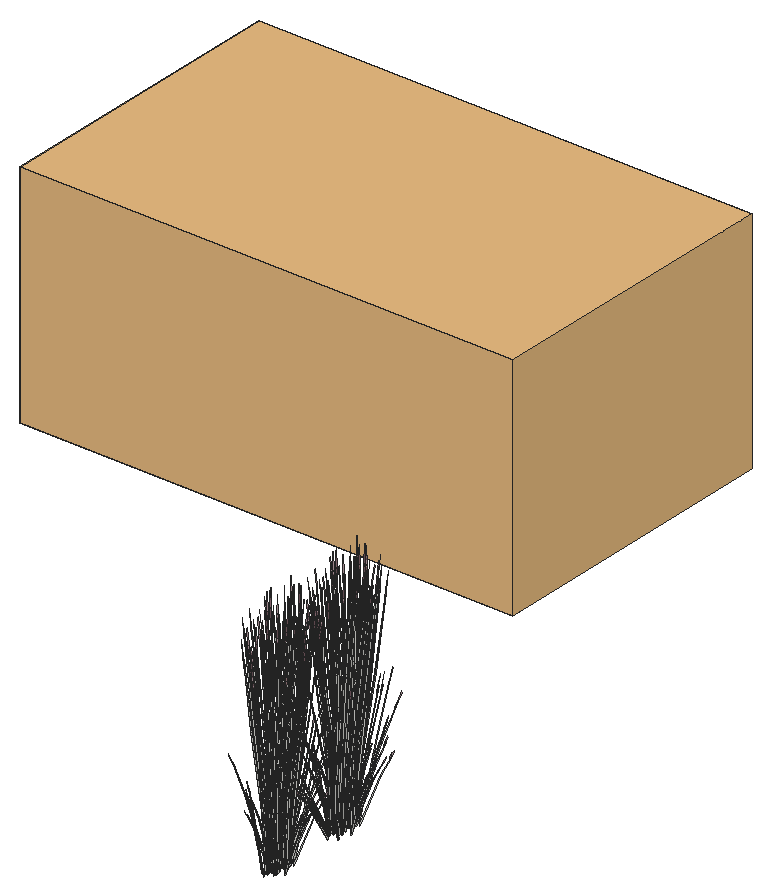
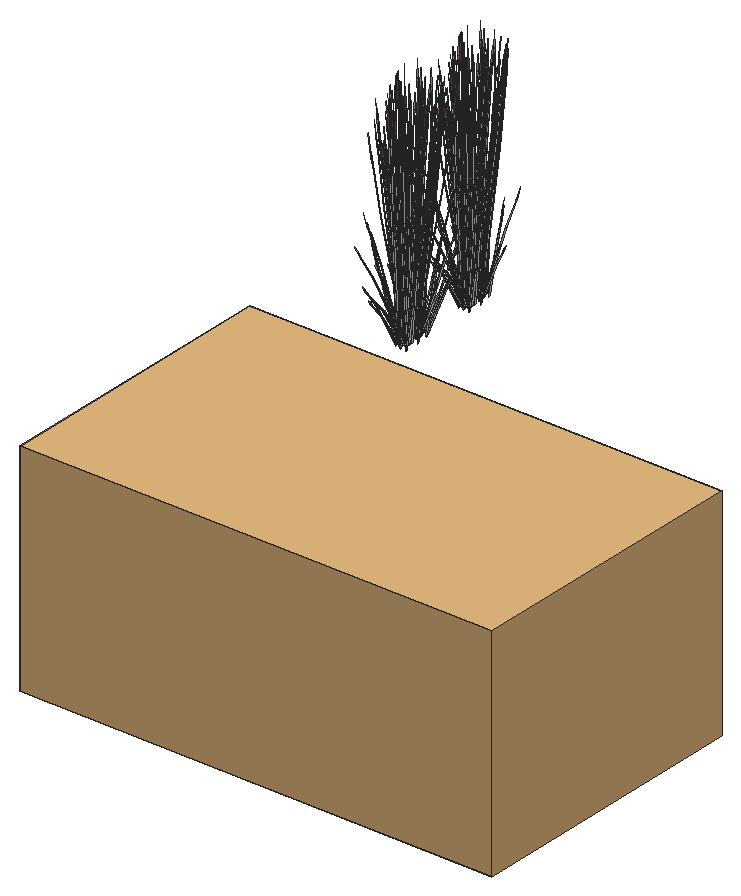
# SketchUp Ruby script. Lengths in inches.
U = 1.inch
M = Sketchup.active_model
def pt(a) = Geom::Point3d.new(a.map { |v| v * U })
def face(e, loops, mat)
  f = e.add_face(loops[0].map { |a| pt(a) })
  loops[1..].each { |l| e.add_face(l.map { |a| pt(a) }).erase! }
  f.material = f.back_material = mat if mat
  f
end
# faces: each face lists its corners as indices into pts; further lists are holes
def faces(e, pts, list, mat = nil) = list.each { |f| face(e, (f[0].is_a?(Array) ? f : [f]).map { |l| l.map { |i| pts[i] } }, mat) }
# xy, xz, yz: faces in a plane at the given z, y or x. An outline is a flat list of corners, or four numbers for a rectangle; further outlines are holes
def ring(l) = l.size == 4 ? [[l[0], l[1]], [l[2], l[1]], [l[2], l[3]], [l[0], l[3]]] : l.each_slice(2).to_a
def flat(e, list, mat, &to3) = list.each { |f| face(e, (f[0].is_a?(Array) ? f : [f]).map { |l| ring(l).map { |u, v| to3.(u, v) } }, mat) }
def xy(e, z, list, mat = nil) = flat(e, list, mat) { |x, y| [x, y, z] }
def xz(e, y, list, mat = nil) = flat(e, list, mat) { |x, z| [x, y, z] }
def yz(e, x, list, mat = nil) = flat(e, list, mat) { |y, z| [x, y, z] }
def lines(e, pts, list) = list.each { |a, b| e.add_line(pt(pts[a]), pt(pts[b])) }
# prism: a flat outline (further loops are holes) pulled along v
def prism(e, loops, v, mat = nil)
  f = face(e, loops, mat); d = Geom::Vector3d.new(v.map { |x| x * U })
  f.pushpull(f.normal.samedirection?(d) ? d.length : -d.length)
end
def box(e, o, s, mat = nil) = prism(e, [[o, [o[0] + s[0], o[1], o[2]], [o[0] + s[0], o[1] + s[1], o[2]], [o[0], o[1] + s[1], o[2]]]], [0, 0, s[2]], mat)
def at(x, y, z, deg = 0) = Geom::Transformation.translation(pt([x, y, z])) * Geom::Transformation.rotation(ORIGIN, Z_AXIS, deg.degrees)
def axes(o, x, y, z) = Geom::Transformation.new([*x, 0, *y, 0, *z, 0, *pt(o).to_a, 1])
def part(name) = M.definitions.add(name)
# library, detail: a bought-in or finely detailed component or shape, given as its bounding box
def library(name, o, s) = part(name).tap { |d| box(d.entities, o, s) }
def detail(e, o, s) = box(e.add_group.entities, o, s)
def put(e, d, t, mat = nil) = e.add_instance(d, t).tap { |i| i.material = mat if mat }
def group(e, t, mat = nil) = e.add_group.tap { |g| g.transformation = t; g.material = mat if mat }.entities
root = M.entities
M.materials.add("LightPink_Translucent").color = [144, 107, 117]
M.materials["LightPink_Translucent"].alpha = 0.75
c1 = part("blade")
p = [[2.15,0.21,22],[0,0.17,0],[0.09,0.45,0],[2.18,0.31,22],[2.29,0.31,22],[0.38,0.45,0],
  [2.48,0.24,33],[2.49,0.24,33],[2.48,0.22,33]]
faces(c1.entities,p,[[0,1,2,3],[4,5,2,3],[6,3,4,7],[8,0,3,6]])
c2 = part("seeds")
p = [[0.3,-0.1,1.38],[-0.01,-0.03,1.59],[-0.01,-0.03,0.03],[0.14,-0.07,-0.07],[0.29,-0.03,3],[0.15,0.01,3.11]]
faces(c2.entities,p,[[0,1,2,3],[1,0,4,5]],"LightPink_Translucent")
c3 = part("blade with seeds")
put(c3.entities,c1,at(0,0,0))
put(c3.entities,c2,axes([2.4,0.25,30.99],[1.5799,-0.05474,1.17369],[-0.12525,1.92788,0.29478],[-0.07173,-0.02425,1.56792]))
c4 = library("2016+Honda+Civic+LX+Sedan",[0.01,0.03,0.02],[16.17,34.46,10.62])
put(root,c3,axes([251.21,225.6,0.91],[-0.16003,-0.61271,0],[0.26773,-0.34169,-0.37456],[0.06098,-0.07782,1.18819]))
put(root,c3,axes([251.56,224.86,0.74],[-0.17688,0.35078,-0.02825],[-0.16207,-0.38418,-0.1281],[-0.01141,-0.10886,0.42251]))
put(root,c3,axes([250.64,227.32,0.66],[0,-0.61145,-0.36036],[0.28637,0,0],[0,-0.13926,1.14313]))
put(root,c3,axes([251.43,225.51,0.66],[0.23955,-0.30573,-0.36036],[0.14318,0.54821,0],[0.05456,-0.06963,1.14313]))
put(root,c3,axes([252.85,226.5625,1.07],[-0.09144,-0.01811,1.03788],[-0.09368,-0.48584,-0.22321],[0.11233,-0.13744,0.44375]))
put(root,c3,axes([251.71,226.76,0.6875],[0.1724,-0.45959,-0.45255],[0.21416,0.41674,-0.11877],[0.06908,-0.11465,0.99892]))
put(root,c3,axes([252.96,225.67,1.2],[-0.08525,0.31126,0.83364],[-0.07328,-0.41819,0.6125],[0.07041,-0.10479,0.18362]))
put(root,c3,axes([251.41,227.57,0.8],[0.12419,-0.55096,-0.32471],[0.25804,0.26516,0.15627],[0,-0.12701,1.04254]))
put(root,c3,axes([251.53,227.29,1.13],[-0.02983,-0.6977,-0.21117],[0.31064,-0.04219,-0.36291],[0.0547,-0.09294,1.15913]))
put(root,c3,axes([250.76,227.33,0.66],[0.17867,-0.3815,-0.22483],[0.17867,0.3815,0.22483],[0,-0.12288,1.00865]))
put(root,c3,axes([250.6875,225.5,0.74],[-0.07384,0.49928,-0.02825],[-0.22725,-0.15358,-0.1281],[-0.0345,-0.08166,0.42251]))
put(root,c3,axes([251.38,228.02,1.13],[-0.28825,-0.29175,-0.21117],[0.1388,-0.61578,-0.36291],[-0.00906,-0.15119,1.15913]))
put(root,c3,axes([250.5625,227.78,0.91],[-0.32006,0,0],[0,-0.68339,-0.37456],[0,-0.15565,1.18819]))
put(root,c3,axes([250.62,226.56,1.07],[0.04997,0.17024,1.03788],[-0.11515,0.46273,-0.22321],[-0.11824,-0.1106,0.44375]))
put(root,c3,axes([251.49,225.75,0.66],[0.23879,0.15129,-0.22483],[-0.06012,0.53279,0.22483],[0.04814,-0.06144,1.00865]))
put(root,c3,axes([250.8125,227.6,0.88],[-0.23808,0.51407,0.22322],[-0.23822,-0.50866,-0.26485],[-0.00831,-0.14599,1.19671]))
put(root,c3,axes([251.57,227.84,0.96],[0.28839,0.29636,0.17466],[-0.1388,0.61578,0.36291],[0,-0.14195,1.16519]))
put(root,c3,axes([251.46,228.67,0.96],[0.06784,-0.72454,-0.17004],[0.32166,0.1263,0.37211],[-0.05621,-0.10006,1.13542]))
put(root,c3,axes([250.32,227.07,1.2],[0.16341,-0.04375,0.83364],[-0.10366,0.38551,0.6125],[-0.08075,-0.05783,0.18362]))
put(root,c3,axes([251.48,227.43,1.17],[-0.27795,0.03775,0.32471],[-0.02514,-0.62656,-0.15627],[0.04976,-0.0635,1.04254]))
put(root,c3,axes([250.76,227.88,0.99],[0,0.61145,0.36036],[-0.28637,0,0],[0,-0.13926,1.14313]))
put(root,c3,axes([252.39,225.76,0.92],[0.16003,-0.61271,0],[0.26773,0.34169,-0.37456],[0.06098,0.07782,1.18819]))
put(root,c3,axes([251.43,228.375,0.8],[-0.15376,-0.51322,-0.32471],[0.2329,-0.3614,0.15627],[-0.04976,-0.0635,1.04254]))
put(root,c3,axes([251.47,227.65,0.91],[0.11128,0.68373,0.33208],[-0.31797,0.23776,0.13031],[0.00389,-0.12563,1.15295]))
put(root,c3,axes([253.02,228.18,0.63],[-0.16485,0.07338,1.02759],[-0.02624,-0.58408,0.05882],[0.11546,-0.08841,0.58473]))
put(root,c3,axes([253.32,227.66,0.83],[-0.15869,-0.39099,-0.04709],[0.1738,-0.35825,-0.21349],[0.04925,-0.02522,0.70419]))
put(root,c3,axes([251.41,228.19,1.17],[-0.12419,0.55096,0.32471],[-0.25804,-0.26516,-0.15627],[0,-0.12701,1.04254]))
put(root,c3,axes([251.87,227.71,0.79],[0,-0.70749,0],[0.32006,0,0],[0,0,1.30246]))
put(root,c3,axes([252.25,226.08,0.99],[-0.23955,-0.30573,0.36036],[0.14318,-0.54821,0],[0.05456,0.06963,1.14313]))
put(root,c3,axes([251.3,228.57,0.6875],[-0.26625,-0.10025,-0.45255],[0.05619,-0.61836,-0.11877],[-0.07946,-0.07493,0.99892]))
put(root,c3,axes([251.71,227.26,0.91],[-0.21222,0.5549,0.33208],[-0.25213,-0.48983,0.13031],[0.05116,-0.05538,1.15295]))
put(root,c3,axes([251.95,228.26,0.86],[-0.23808,-0.52628,-0.0445],[0.23822,-0.5266,0],[-0.00831,-0.01838,1.27426]))
put(root,c3,axes([251.35,226.35,0.99],[-0.07394,0.60768,0.12804],[-0.27057,-0.17197,0.25465],[0.04674,-0.00296,1.1642]))
put(root,c3,axes([251.23,226.84,0.35],[-0.25194,0.2448,0.93574],[-0.08019,-0.7024,0.36359],[0.1547,0.01169,1.0643]))
put(root,c3,axes([251.91,227.03,1.09],[0.04938,-0.54569,0.10509],[0.24125,0.09472,-0.30009],[0.0439,0.05603,0.91989]))
put(root,c3,axes([251.49,228.32,0.91],[0.32351,0.12883,0.33208],[-0.06584,0.72759,0.13031],[-0.04728,-0.07026,1.15295]))
put(root,c3,axes([253.2,227.79,0.28],[-0.01338,-0.09283,1.27986],[0.09278,-0.54301,-0.19552],[0.09359,-0.00781,0.218]))
put(root,c3,axes([250.44,227.7,0.28],[0.00649,0.09636,1.27986],[-0.13086,0.50324,-0.19552],[-0.09295,-0.02537,0.218]))
put(root,c3,axes([251.81,227.17,1.17],[-0.15376,-0.51322,0.32471],[0.2329,-0.3614,-0.15627],[0.04976,0.0635,1.04254]))
put(root,c3,axes([251.01,229.52,0.66],[-0.06012,-0.53279,-0.22483],[0.23879,-0.15129,0.22483],[-0.04814,-0.06144,1.00865]))
put(root,c3,axes([251.32,229.48,0.99],[0.27504,-0.16229,0.12804],[0.06792,0.60396,0.25465],[-0.02453,-0.088,1.1642]))
put(root,c3,axes([251.89,227.2,1.13],[0.25843,-0.40595,-0.21117],[0.17185,0.5736,-0.36291],[0.06376,0.05825,1.15913]))
put(root,c3,axes([250.95,229.74,0.66],[-0.23955,-0.30573,-0.36036],[0.14318,-0.54821,0],[-0.05456,-0.06963,1.14313]))
put(root,c3,axes([252.54,226.125,0.66],[0.23955,0.30573,-0.36036],[-0.14318,0.54821,0],[0.05456,0.06963,1.14313]))
put(root,c3,axes([252.08,227.87,0.79],[0.28637,0,0],[0,0.63302,0],[0,0,1.29484]))
put(root,c3,axes([251.6,228.66,1.13],[-0.25843,0.40595,-0.21117],[-0.17185,-0.5736,-0.36291],[-0.06376,-0.05825,1.15913]))
put(root,c3,axes([252.16,226.38,0.99],[-0.27504,0.16229,0.12804],[-0.06792,-0.60396,0.25465],[0.02453,0.088,1.1642]))
put(root,c3,axes([252.47,226.35,0.66],[0.06012,0.53279,-0.22483],[-0.23879,0.15129,0.22483],[0.04814,0.06144,1.00865]))
put(root,c3,axes([251.99,227.55,0.92],[-0.32351,-0.12883,0.35707],[0.06584,-0.72759,0.14012],[0.04728,0.07026,1.23973]))
put(root,c3,axes([251.73,229.34,0.79],[-0.08351,-0.52716,0],[0.23848,-0.18461,0],[0,0,1.1204]))
put(root,c3,axes([251.57,228.84,1.09],[-0.04938,0.54569,0.10509],[-0.24125,-0.09472,-0.30009],[-0.0439,-0.05603,0.91989]))
put(root,c3,axes([252.05,229.27,0.78],[0.26872,-0.20746,-0.13933],[0.09442,0.59762,0.00006],[0.02966,-0.02293,1.26212]))
put(root,c3,axes([252.14,229.52,0.99],[0.07394,-0.60768,0.12804],[0.27057,0.17197,0.25465],[-0.04674,0.00296,1.1642]))
put(root,c3,axes([252.08,228.14,0.8],[0.17867,0.39495,0],[-0.17867,0.39495,0],[0,0,1.22851]))
put(root,c3,axes([252.5625,227.97,0.99],[-0.2011,-0.44539,0.12804],[0.20266,-0.432,0.25465],[-0.02221,0.09096,1.1642]))
put(root,c3,axes([252.1875,227.29,0.6875],[0.26625,0.10025,-0.45255],[-0.05619,0.61836,-0.11877],[0.07946,0.07493,0.99892]))
put(root,c3,axes([253.36,228.375,1.2],[-0.15814,0.10094,0.83364],[0.07444,-0.41719,0.6125],[0.0839,0.02855,0.18362]))
put(root,c3,axes([251.67,229.58,0.79],[-0.25804,-0.27452,0],[0.12419,-0.5704,0],[0,0,1.1809]))
put(root,c3,axes([251.89,228.85,0.98],[-0.24993,-0.49214,-0.18284],[0.21031,-0.55263,0.40012],[-0.0673,0.05757,1.22088]))
put(root,c3,axes([251.23,229.79,0.99],[0.23955,0.30573,0.36036],[-0.14318,0.54821,0],[-0.05456,-0.06963,1.14313]))
put(root,c3,axes([252.07,227.68,1.17],[0.12419,-0.55096,0.32471],[0.25804,0.26516,-0.15627],[0,0.12701,1.04254]))
put(root,c3,axes([252.03,227.99,0.86],[0,0.70714,-0.04091],[-0.32006,0,0],[0,0.02222,1.30182]))
put(root,c3,axes([252.05,227.49,0.8],[0.15376,0.51322,-0.32471],[-0.2329,0.3614,0.15627],[0.04976,0.0635,1.04254]))
put(root,c3,axes([251.09,230.11,0.91],[-0.16003,0.61271,0],[-0.26773,-0.34169,-0.37456],[-0.06098,-0.07782,1.18819]))
put(root,c3,axes([252.73,227.98,0.99],[0,-0.61145,0.36036],[0.28637,0,0],[0,0.13926,1.14313]))
put(root,c3,axes([252.01,228.44,1.17],[0.27795,-0.03775,0.32471],[0.02514,0.62656,-0.15627],[-0.04976,0.0635,1.04254]))
put(root,c3,axes([252.18,227.8,1.09],[0.23848,-0.17832,0.10509],[0.08351,0.5092,-0.30009],[0,0.11207,0.91989]))
put(root,c3,axes([251.76,228.75,0.8],[-0.27795,0.03775,-0.32471],[-0.02514,-0.62656,0.15627],[-0.04976,0.0635,1.04254]))
put(root,c3,axes([253.07,229.04,1.07],[-0.06164,-0.15038,1.03788],[0.0802,-0.49748,-0.22321],[0.12472,0.06739,0.44375]))
put(root,c3,axes([251.97,229.59,0.79],[0.25804,0.27452,0],[-0.12419,0.5704,0],[0,0,1.26978]))
put(root,c3,axes([252.07,230.2,0.78],[-0.15803,-0.61485,-0.03732],[0.26773,-0.34169,0.37456],[-0.06597,0.05854,1.1876]))
put(root,c3,axes([252.01,228.71,1.09],[0.1891,0.36737,0.10509],[-0.15773,0.41447,-0.30009],[-0.0439,0.05603,0.91989]))
put(root,c3,axes([252.21,229.84,0.99],[0.23955,-0.30573,0.36036],[0.14318,0.54821,0],[-0.05456,0.06963,1.14313]))
put(root,c3,axes([251.875,229.36,0.86],[0.11128,0.70245,-0.04364],[-0.31797,0.24614,0],[0.00389,0.02453,1.2496]))
put(root,c3,axes([252,230.12,0.66],[-0.23879,-0.15129,-0.22483],[0.06012,-0.53279,0.22483],[-0.04814,0.06144,1.00865]))
put(root,c3,axes([250.27,229.04,1.07],[0.08895,0.05019,1.03788],[0.05733,0.5127,-0.22321],[-0.12083,0.09597,0.44375]))
put(root,c3,axes([252.92,228.09,0.92],[0.32006,0,0],[0,0.68339,-0.37456],[0,0.15565,1.18819]))
put(root,c3,axes([252.79,228.4375,0.79],[-0.3199,-0.00489,-0.03612],[0,-0.68339,0.36248],[-0.01005,0.15557,1.14929]))
put(root,c3,axes([252.1,227.84,1.13],[0.28825,0.29175,-0.21117],[-0.1388,0.61578,-0.36291],[0.00906,0.15119,1.15913]))
put(root,c3,axes([250.09,230.11,1.2],[0.10667,-0.27712,0.83364],[0.04209,0.43871,0.6125],[-0.07709,0.07855,0.18362]))
put(root,c3,axes([252.73,228.54,0.66],[-0.17867,0.3815,-0.22483],[-0.17867,-0.3815,0.22483],[0,0.12288,1.00865]))
put(root,c3,axes([251.96,228.58,1.13],[0.02983,0.6977,-0.21117],[-0.31064,0.04219,-0.36291],[-0.0547,0.09294,1.15913]))
put(root,c3,axes([252.07,228.3,0.8],[-0.12419,0.55096,-0.32471],[-0.25804,-0.26516,0.15627],[0,0.12701,1.04254]))
put(root,c3,axes([251.77,229.11,0.6875],[-0.1724,0.45959,-0.45255],[-0.21416,-0.41674,-0.11877],[-0.06908,0.11465,0.99892]))
put(root,c3,axes([252.08,229.88,0.88],[0.32044,0.19874,0.22322],[-0.08017,0.71038,-0.26485],[-0.05304,0.08891,1.19671]))
put(root,c3,axes([252.05,230.36,0.66],[-0.23955,0.30573,-0.36036],[-0.14318,-0.54821,0],[-0.05456,0.06963,1.14313]))
put(root,c3,axes([252.85,228.55,0.66],[0,0.61145,-0.36036],[-0.28637,0,0],[0,0.13926,1.14313]))
put(root,c3,axes([252.49,229.82,1.2],[-0.14411,-0.17581,0.83364],[0.18609,-0.17864,0.6125],[0.05019,0.15132,0.18362]))
put(root,c3,axes([252.27,230.27,0.91],[0.16003,0.61271,0],[-0.26773,0.34169,-0.37456],[-0.06098,0.07782,1.18819]))
put(root,c3,axes([252.53,230.47,0.28],[0.01865,-0.08828,1.27986],[0.23477,-0.25998,-0.19552],[0.07118,0.13456,0.218]))
put(root,c3,axes([252.13,227.84,1.26],[-0.00699,-0.5757,1.02533],[0.31645,0.14923,0.43413],[-0.07484,0.31502,0.96783]))
put(root,c3,axes([252.22,228.47,0.71],[0.09385,0.55983,-0.50233],[-0.27035,0.20162,-0.13184],[0.01037,0.18957,1.1088]))
put(root,c3,axes([250.37,230.4,0.28],[0.03433,0.06109,1.27986],[0.05822,0.56601,-0.19552],[-0.07609,0.1207,0.218]))
put(root,c3,axes([252.51,230.62,1.13],[-0.16414,-0.01918,0.76251],[0.10839,-0.40729,0.421],[0.06484,0.1447,0.59812]))
put(root,c3,axes([251.97,229.63,1.07],[0.00452,-0.20269,1.03788],[0.21585,-0.22641,-0.22321],[0.06663,0.2426,0.44375]))
put(root,c3,axes([250.99,231.32,1.2],[-0.00662,-0.36357,0.83364],[0.16552,0.25931,0.6125],[-0.03255,0.17329,0.18362]))
put(root,c3,axes([251.43,230.45,0.28],[0.04142,-0.03327,1.27986],[0.24917,0.18313,-0.19552],[0.00729,0.2064,0.218]))
put(root,c3,axes([250.86,230.54,1.24],[0.23252,-0.10828,0.04723],[0.05346,0.43623,-0.62638],[-0.01474,0.22082,0.56147]))
put(root,c3,axes([252.15,240.19,1.07],[-0.07276,0.12376,1.03788],[-0.21789,-0.21662,-0.22321],[0.04039,-0.2694,0.44375]))
put(root,c3,axes([250.8,231,1.07],[0.08077,-0.09646,1.03788],[0.19942,0.29084,-0.22321],[-0.05936,0.25166,0.44375]))
put(root,c3,axes([251.03,239.96,1.07],[-0.0155,0.20002,1.03788],[-0.22659,0.16744,-0.22321],[-0.05297,-0.25854,0.44375]))
put(root,c3,axes([251.61,239.52,0.28],[-0.04293,0.02203,1.27986],[-0.23742,-0.24798,-0.19552],[0.00398,-0.20684,0.218]))
put(root,c3,axes([251.88,239.2,1.2],[0.03283,0.35655,0.83364],[-0.18215,-0.19748,0.6125],[0.0196,-0.18257,0.18362]))
put(root,c3,axes([250.95,239.63,1.2],[0.13352,0.21281,0.83364],[-0.19445,0.12793,0.6125],[-0.0416,-0.16355,0.18362]))
put(root,c3,axes([250.84,240.27,0.28],[-0.02479,0.08055,1.27986],[-0.25056,0.17367,-0.19552],[-0.06053,-0.15798,0.218]))
put(root,c3,axes([251.25,242.49,0.72],[-0.10512,-0.62701,-0.50685],[0.30279,-0.22582,-0.13303],[-0.01162,-0.21232,1.11879]))
put(root,c3,axes([252.66,240.57,0.28],[-0.03831,-0.04817,1.27986],[-0.0984,-0.53815,-0.19552],[0.06638,-0.14604,0.218]))
put(root,c3,axes([251.21,240.69,0.91],[-0.16003,-0.61271,0],[0.26773,-0.34169,-0.37456],[0.06098,-0.07782,1.18819]))
put(root,c3,axes([251.56,239.95,0.74],[-0.17688,0.35078,-0.02825],[-0.16207,-0.38418,-0.1281],[-0.01141,-0.10886,0.42251]))
put(root,c3,axes([250.64,242.4,0.66],[0,-0.61145,-0.36036],[0.28637,0,0],[0,-0.13926,1.14313]))
put(root,c3,axes([251.43,240.59,0.66],[0.23955,-0.30573,-0.36036],[0.14318,0.54821,0],[0.05456,-0.06963,1.14313]))
put(root,c3,axes([252.85,241.65,1.07],[-0.09144,-0.01811,1.03788],[-0.09368,-0.48584,-0.22321],[0.11233,-0.13744,0.44375]))
put(root,c3,axes([251.71,241.84,0.6875],[0.1724,-0.45959,-0.45255],[0.21416,0.41674,-0.11877],[0.06908,-0.11465,0.99892]))
put(root,c3,axes([252.96,240.75,1.2],[-0.08525,0.31126,0.83364],[-0.07328,-0.41819,0.6125],[0.07041,-0.10479,0.18362]))
put(root,c3,axes([251.41,242.65,0.8],[0.12419,-0.55096,-0.32471],[0.25804,0.26516,0.15627],[0,-0.12701,1.04254]))
put(root,c3,axes([251.53,242.375,1.13],[-0.02983,-0.6977,-0.21117],[0.31064,-0.04219,-0.36291],[0.0547,-0.09294,1.15913]))
put(root,c3,axes([250.76,242.41,0.66],[0.17867,-0.3815,-0.22483],[0.17867,0.3815,0.22483],[0,-0.12288,1.00865]))
put(root,c3,axes([250.6875,240.58,0.74],[-0.07384,0.49928,-0.02825],[-0.22725,-0.15358,-0.1281],[-0.0345,-0.08166,0.42251]))
put(root,c3,axes([251.38,243.11,1.13],[-0.28825,-0.29175,-0.21117],[0.1388,-0.61578,-0.36291],[-0.00906,-0.15119,1.15913]))
put(root,c3,axes([250.5625,242.86,0.91],[-0.32006,0,0],[0,-0.68339,-0.37456],[0,-0.15565,1.18819]))
put(root,c3,axes([250.62,241.64,1.07],[0.04997,0.17024,1.03788],[-0.11515,0.46273,-0.22321],[-0.11824,-0.1106,0.44375]))
put(root,c3,axes([251.49,240.83,0.66],[0.23879,0.15129,-0.22483],[-0.06012,0.53279,0.22483],[0.04814,-0.06144,1.00865]))
put(root,c3,axes([250.8125,242.68,0.88],[-0.23808,0.51407,0.22322],[-0.23822,-0.50866,-0.26485],[-0.00831,-0.14599,1.19671]))
put(root,c3,axes([251.57,242.92,0.96],[0.28839,0.29636,0.17466],[-0.1388,0.61578,0.36291],[0,-0.14195,1.16519]))
put(root,c3,axes([251.46,243.76,0.96],[0.06784,-0.72454,-0.17004],[0.32166,0.1263,0.37211],[-0.05621,-0.10006,1.13542]))
put(root,c3,axes([250.32,242.15,1.2],[0.16341,-0.04375,0.83364],[-0.10366,0.38551,0.6125],[-0.08075,-0.05783,0.18362]))
put(root,c3,axes([251.48,242.51,1.17],[-0.27795,0.03775,0.32471],[-0.02514,-0.62656,-0.15627],[0.04976,-0.0635,1.04254]))
put(root,c3,axes([250.76,242.97,0.99],[0,0.61145,0.36036],[-0.28637,0,0],[0,-0.13926,1.14313]))
put(root,c3,axes([252.39,240.84,0.92],[0.16003,-0.61271,0],[0.26773,0.34169,-0.37456],[0.06098,0.07782,1.18819]))
put(root,c3,axes([251.43,243.46,0.8],[-0.15376,-0.51322,-0.32471],[0.2329,-0.3614,0.15627],[-0.04976,-0.0635,1.04254]))
put(root,c3,axes([251.47,242.74,0.91],[0.11128,0.68373,0.33208],[-0.31797,0.23776,0.13031],[0.00389,-0.12563,1.15295]))
put(root,c3,axes([253.02,243.26,0.63],[-0.16485,0.07338,1.02759],[-0.02624,-0.58408,0.05882],[0.11546,-0.08841,0.58473]))
put(root,c3,axes([253.32,242.74,0.83],[-0.15869,-0.39099,-0.04709],[0.1738,-0.35825,-0.21349],[0.04925,-0.02522,0.70419]))
put(root,c3,axes([251.41,243.28,1.17],[-0.12419,0.55096,0.32471],[-0.25804,-0.26516,-0.15627],[0,-0.12701,1.04254]))
put(root,c3,axes([251.87,242.79,0.79],[0,-0.70749,0],[0.32006,0,0],[0,0,1.30246]))
put(root,c3,axes([252.25,241.16,0.99],[-0.23955,-0.30573,0.36036],[0.14318,-0.54821,0],[0.05456,0.06963,1.14313]))
put(root,c3,axes([251.3,243.66,0.6875],[-0.26625,-0.10025,-0.45255],[0.05619,-0.61836,-0.11877],[-0.07946,-0.07493,0.99892]))
put(root,c3,axes([251.71,242.35,0.91],[-0.21222,0.5549,0.33208],[-0.25213,-0.48983,0.13031],[0.05116,-0.05538,1.15295]))
put(root,c3,axes([251.95,243.34,0.86],[-0.23808,-0.52628,-0.0445],[0.23822,-0.5266,0],[-0.00831,-0.01838,1.27426]))
put(root,c3,axes([251.35,241.43,0.99],[-0.07394,0.60768,0.12804],[-0.27057,-0.17197,0.25465],[0.04674,-0.00296,1.1642]))
put(root,c3,axes([251.23,241.93,0.35],[-0.25194,0.2448,0.93574],[-0.08019,-0.7024,0.36359],[0.1547,0.01169,1.0643]))
put(root,c3,axes([251.91,242.11,1.09],[0.04938,-0.54569,0.10509],[0.24125,0.09472,-0.30009],[0.0439,0.05603,0.91989]))
put(root,c3,axes([251.49,243.41,0.91],[0.32351,0.12883,0.33208],[-0.06584,0.72759,0.13031],[-0.04728,-0.07026,1.15295]))
put(root,c3,axes([253.2,242.88,0.28],[-0.01338,-0.09283,1.27986],[0.09278,-0.54301,-0.19552],[0.09359,-0.00781,0.218]))
put(root,c3,axes([250.44,242.78,0.28],[0.00649,0.09636,1.27986],[-0.13086,0.50324,-0.19552],[-0.09295,-0.02537,0.218]))
put(root,c3,axes([251.81,242.25,1.17],[-0.15376,-0.51322,0.32471],[0.2329,-0.3614,-0.15627],[0.04976,0.0635,1.04254]))
put(root,c3,axes([251.01,244.6,0.66],[-0.06012,-0.53279,-0.22483],[0.23879,-0.15129,0.22483],[-0.04814,-0.06144,1.00865]))
put(root,c3,axes([251.32,244.57,0.99],[0.27504,-0.16229,0.12804],[0.06792,0.60396,0.25465],[-0.02453,-0.088,1.1642]))
put(root,c3,axes([251.89,242.29,1.13],[0.25843,-0.40595,-0.21117],[0.17185,0.5736,-0.36291],[0.06376,0.05825,1.15913]))
put(root,c3,axes([250.95,244.83,0.66],[-0.23955,-0.30573,-0.36036],[0.14318,-0.54821,0],[-0.05456,-0.06963,1.14313]))
put(root,c3,axes([252.54,241.21,0.66],[0.23955,0.30573,-0.36036],[-0.14318,0.54821,0],[0.05456,0.06963,1.14313]))
put(root,c3,axes([252.08,242.95,0.79],[0.28637,0,0],[0,0.63302,0],[0,0,1.29484]))
put(root,c3,axes([251.6,243.75,1.13],[-0.25843,0.40595,-0.21117],[-0.17185,-0.5736,-0.36291],[-0.06376,-0.05825,1.15913]))
put(root,c3,axes([252.16,241.47,0.99],[-0.27504,0.16229,0.12804],[-0.06792,-0.60396,0.25465],[0.02453,0.088,1.1642]))
put(root,c3,axes([252.47,241.4375,0.66],[0.06012,0.53279,-0.22483],[-0.23879,0.15129,0.22483],[0.04814,0.06144,1.00865]))
put(root,c3,axes([251.99,242.63,0.92],[-0.32351,-0.12883,0.35707],[0.06584,-0.72759,0.14012],[0.04728,0.07026,1.23973]))
put(root,c3,axes([251.73,244.43,0.79],[-0.08351,-0.52716,0],[0.23848,-0.18461,0],[0,0,1.1204]))
put(root,c3,axes([251.57,243.93,1.09],[-0.04938,0.54569,0.10509],[-0.24125,-0.09472,-0.30009],[-0.0439,-0.05603,0.91989]))
put(root,c3,axes([252.05,244.35,0.78],[0.26872,-0.20746,-0.13933],[0.09442,0.59762,0.00006],[0.02966,-0.02293,1.26212]))
put(root,c3,axes([252.14,244.6,0.99],[0.07394,-0.60768,0.12804],[0.27057,0.17197,0.25465],[-0.04674,0.00296,1.1642]))
put(root,c3,axes([252.08,243.22,0.8],[0.17867,0.39495,0],[-0.17867,0.39495,0],[0,0,1.22851]))
put(root,c3,axes([252.5625,243.05,0.99],[-0.2011,-0.44539,0.12804],[0.20266,-0.432,0.25465],[-0.02221,0.09096,1.1642]))
put(root,c3,axes([252.1875,242.38,0.6875],[0.26625,0.10025,-0.45255],[-0.05619,0.61836,-0.11877],[0.07946,0.07493,0.99892]))
put(root,c3,axes([253.36,243.46,1.2],[-0.15814,0.10094,0.83364],[0.07444,-0.41719,0.6125],[0.0839,0.02855,0.18362]))
put(root,c3,axes([251.67,244.67,0.79],[-0.25804,-0.27452,0],[0.12419,-0.5704,0],[0,0,1.1809]))
put(root,c3,axes([251.89,243.93,0.98],[-0.24993,-0.49214,-0.18284],[0.21031,-0.55263,0.40012],[-0.0673,0.05757,1.22088]))
put(root,c3,axes([251.23,244.88,0.99],[0.23955,0.30573,0.36036],[-0.14318,0.54821,0],[-0.05456,-0.06963,1.14313]))
put(root,c3,axes([252.07,242.76,1.17],[0.12419,-0.55096,0.32471],[0.25804,0.26516,-0.15627],[0,0.12701,1.04254]))
put(root,c3,axes([252.03,243.08,0.86],[0,0.70714,-0.04091],[-0.32006,0,0],[0,0.02222,1.30182]))
put(root,c3,axes([252.05,242.58,0.8],[0.15376,0.51322,-0.32471],[-0.2329,0.3614,0.15627],[0.04976,0.0635,1.04254]))
put(root,c3,axes([251.09,245.2,0.91],[-0.16003,0.61271,0],[-0.26773,-0.34169,-0.37456],[-0.06098,-0.07782,1.18819]))
put(root,c3,axes([252.73,243.07,0.99],[0,-0.61145,0.36036],[0.28637,0,0],[0,0.13926,1.14313]))
put(root,c3,axes([252.01,243.53,1.17],[0.27795,-0.03775,0.32471],[0.02514,0.62656,-0.15627],[-0.04976,0.0635,1.04254]))
put(root,c3,axes([252.18,242.89,1.09],[0.23848,-0.17832,0.10509],[0.08351,0.5092,-0.30009],[0,0.11207,0.91989]))
put(root,c3,axes([251.76,243.83,0.8],[-0.27795,0.03775,-0.32471],[-0.02514,-0.62656,0.15627],[-0.04976,0.0635,1.04254]))
put(root,c3,axes([253.07,244.13,1.07],[-0.06164,-0.15038,1.03788],[0.0802,-0.49748,-0.22321],[0.12472,0.06739,0.44375]))
put(root,c3,axes([251.97,244.68,0.79],[0.25804,0.27452,0],[-0.12419,0.5704,0],[0,0,1.26978]))
put(root,c3,axes([252.07,245.28,0.78],[-0.15803,-0.61485,-0.03732],[0.26773,-0.34169,0.37456],[-0.06597,0.05854,1.1876]))
put(root,c3,axes([252.01,243.8,1.09],[0.1891,0.36737,0.10509],[-0.15773,0.41447,-0.30009],[-0.0439,0.05603,0.91989]))
put(root,c3,axes([252.21,244.93,0.99],[0.23955,-0.30573,0.36036],[0.14318,0.54821,0],[-0.05456,0.06963,1.14313]))
put(root,c3,axes([251.875,244.45,0.86],[0.11128,0.70245,-0.04364],[-0.31797,0.24614,0],[0.00389,0.02453,1.2496]))
put(root,c3,axes([252,245.2,0.66],[-0.23879,-0.15129,-0.22483],[0.06012,-0.53279,0.22483],[-0.04814,0.06144,1.00865]))
put(root,c3,axes([250.27,244.125,1.07],[0.08895,0.05019,1.03788],[0.05733,0.5127,-0.22321],[-0.12083,0.09597,0.44375]))
put(root,c3,axes([252.92,243.17,0.92],[0.32006,0,0],[0,0.68339,-0.37456],[0,0.15565,1.18819]))
put(root,c3,axes([252.79,243.52,0.79],[-0.3199,-0.00489,-0.03612],[0,-0.68339,0.36248],[-0.01005,0.15557,1.14929]))
put(root,c3,axes([252.1,242.93,1.13],[0.28825,0.29175,-0.21117],[-0.1388,0.61578,-0.36291],[0.00906,0.15119,1.15913]))
put(root,c3,axes([250.09,245.2,1.2],[0.10667,-0.27712,0.83364],[0.04209,0.43871,0.6125],[-0.07709,0.07855,0.18362]))
put(root,c3,axes([252.73,243.625,0.66],[-0.17867,0.3815,-0.22483],[-0.17867,-0.3815,0.22483],[0,0.12288,1.00865]))
put(root,c3,axes([251.96,243.66,1.13],[0.02983,0.6977,-0.21117],[-0.31064,0.04219,-0.36291],[-0.0547,0.09294,1.15913]))
put(root,c3,axes([252.07,243.39,0.8],[-0.12419,0.55096,-0.32471],[-0.25804,-0.26516,0.15627],[0,0.12701,1.04254]))
put(root,c3,axes([251.77,244.19,0.6875],[-0.1724,0.45959,-0.45255],[-0.21416,-0.41674,-0.11877],[-0.06908,0.11465,0.99892]))
put(root,c3,axes([252.08,244.97,0.88],[0.32044,0.19874,0.22322],[-0.08017,0.71038,-0.26485],[-0.05304,0.08891,1.19671]))
put(root,c3,axes([252.05,245.45,0.66],[-0.23955,0.30573,-0.36036],[-0.14318,-0.54821,0],[-0.05456,0.06963,1.14313]))
put(root,c3,axes([252.85,243.64,0.66],[0,0.61145,-0.36036],[-0.28637,0,0],[0,0.13926,1.14313]))
put(root,c3,axes([252.49,244.91,1.2],[-0.14411,-0.17581,0.83364],[0.18609,-0.17864,0.6125],[0.05019,0.15132,0.18362]))
put(root,c3,axes([252.27,245.35,0.91],[0.16003,0.61271,0],[-0.26773,0.34169,-0.37456],[-0.06098,0.07782,1.18819]))
put(root,c3,axes([252.53,245.56,0.28],[0.01865,-0.08828,1.27986],[0.23477,-0.25998,-0.19552],[0.07118,0.13456,0.218]))
put(root,c3,axes([252.13,242.93,1.26],[-0.00699,-0.5757,1.02533],[0.31645,0.14923,0.43413],[-0.07484,0.31502,0.96783]))
put(root,c3,axes([252.22,243.55,0.71],[0.09385,0.55983,-0.50233],[-0.27035,0.20162,-0.13184],[0.01037,0.18957,1.1088]))
put(root,c3,axes([250.37,245.48,0.28],[0.03433,0.06109,1.27986],[0.05822,0.56601,-0.19552],[-0.07609,0.1207,0.218]))
put(root,c3,axes([252.51,245.71,1.13],[-0.16414,-0.01918,0.76251],[0.10839,-0.40729,0.421],[0.06484,0.1447,0.59812]))
put(root,c3,axes([251.97,244.72,1.07],[0.00452,-0.20269,1.03788],[0.21585,-0.22641,-0.22321],[0.06663,0.2426,0.44375]))
put(root,c3,axes([250.99,246.41,1.2],[-0.00662,-0.36357,0.83364],[0.16552,0.25931,0.6125],[-0.03255,0.17329,0.18362]))
put(root,c3,axes([251.43,245.54,0.28],[0.04142,-0.03327,1.27986],[0.24917,0.18313,-0.19552],[0.00729,0.2064,0.218]))
put(root,c3,axes([250.86,245.62,1.24],[0.23252,-0.10828,0.04723],[0.05346,0.43623,-0.62638],[-0.01474,0.22082,0.56147]))
put(root,c3,axes([250.8,246.08,1.07],[0.08077,-0.09646,1.03788],[0.19942,0.29084,-0.22321],[-0.05936,0.25166,0.44375]))
put(root,c4,axes([140.4375,362.48,-0.09],[0,-3.39415,0],[2.62357,0,0],[0,0,3.9591]))
